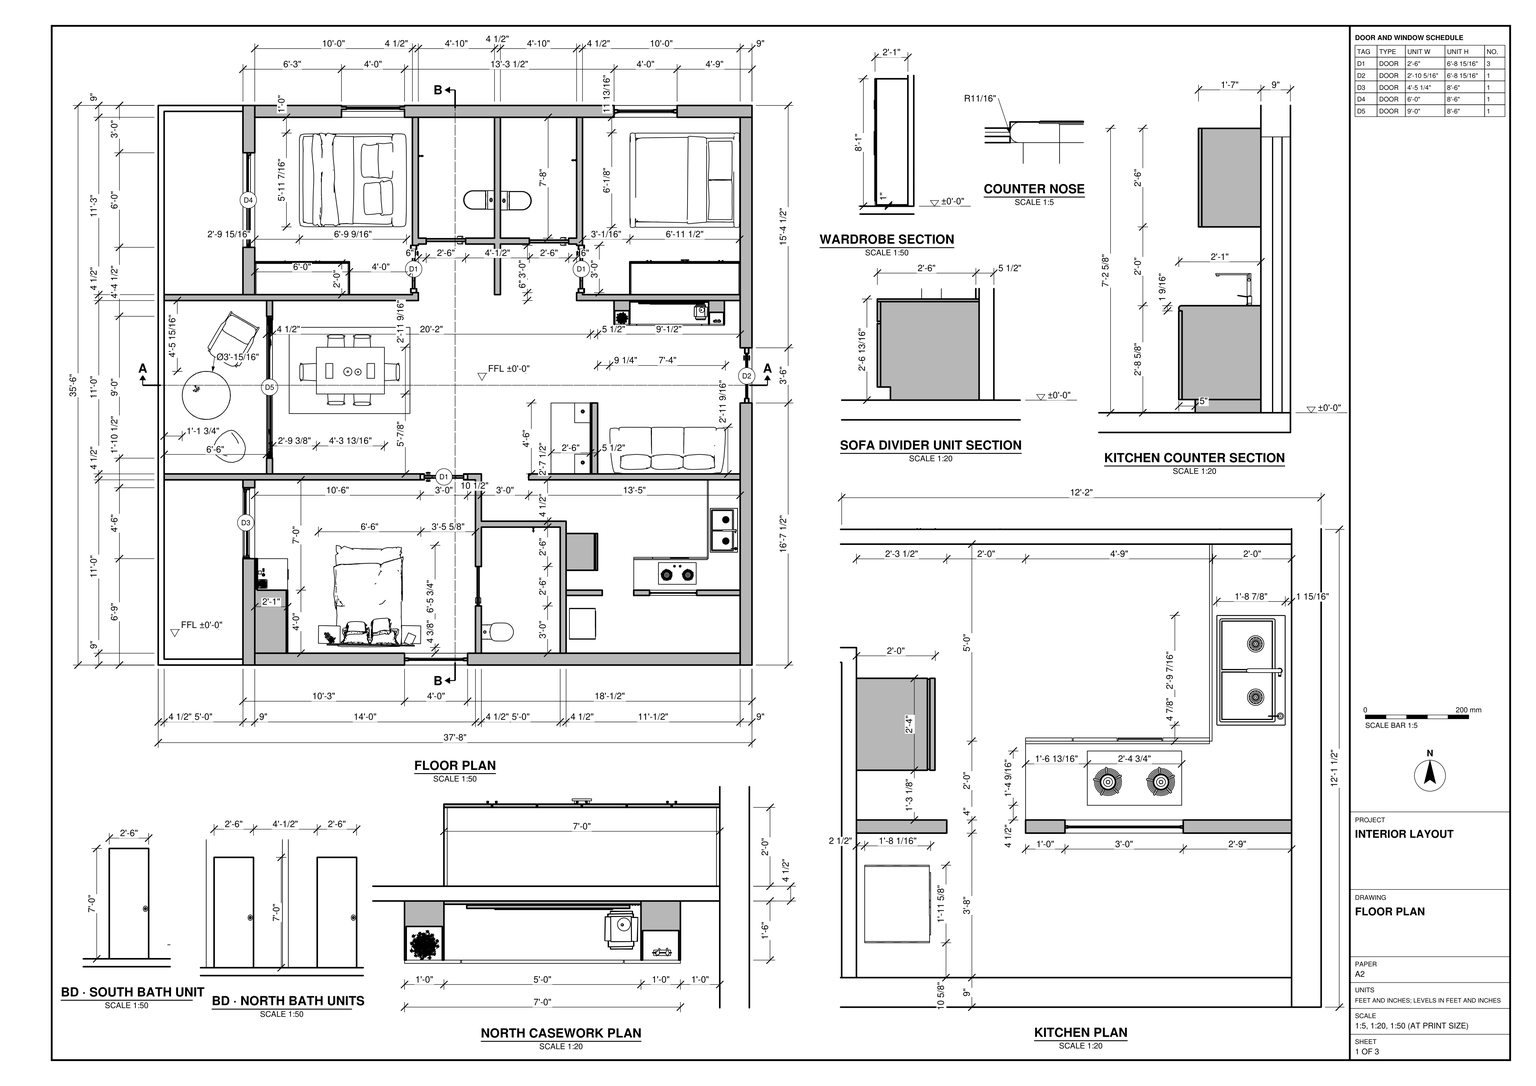
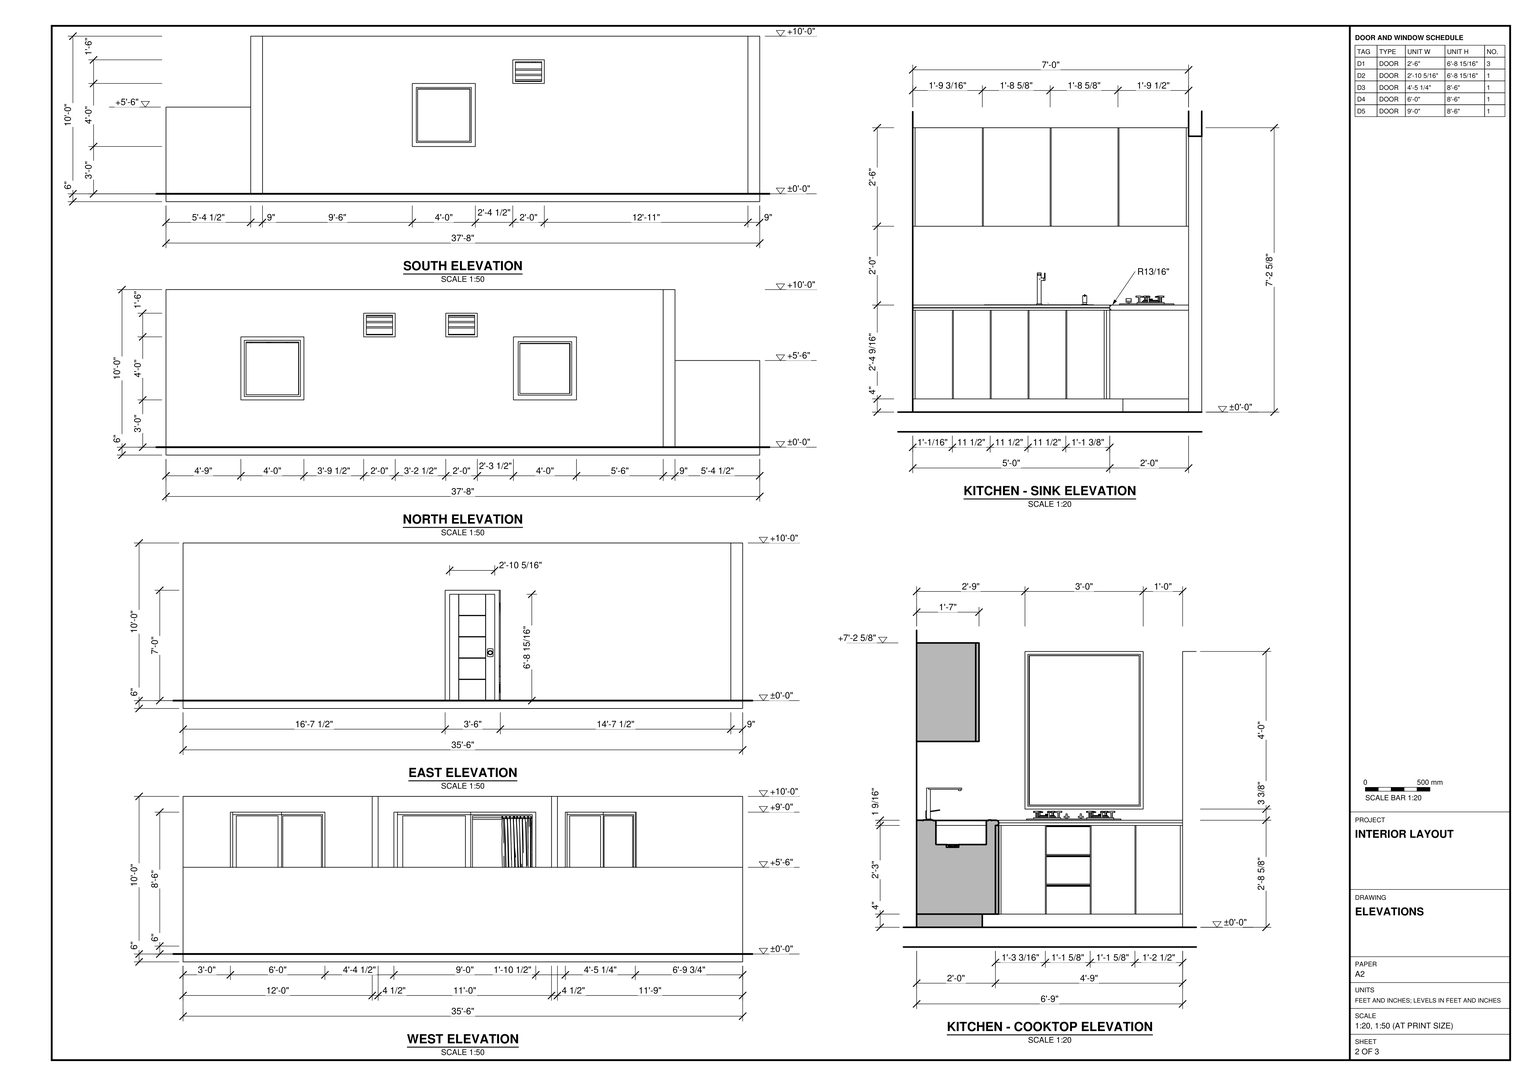
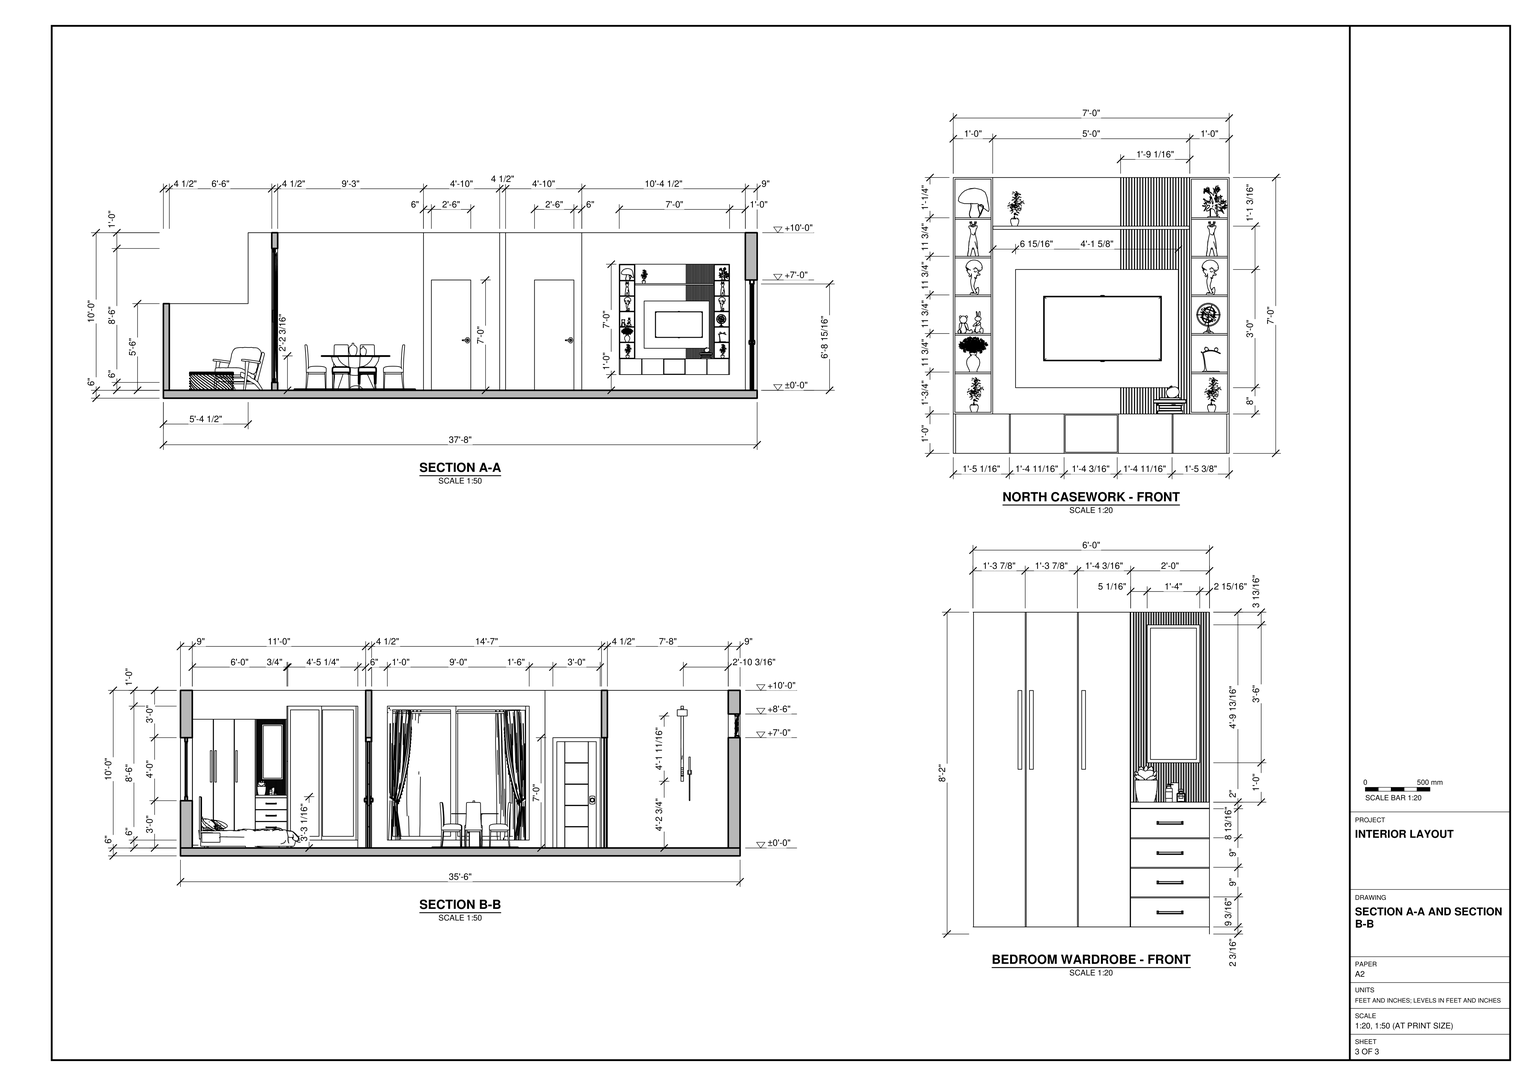
Build the residential interior in SketchUp from task_files/diagram_01.pdf. Work in feet and inches. Set the single finished floor at ±0'-0". The overall model shall measure 37'-8" east to west, 35'-6" north to south and 10'-6" from the underside of the slab to the top of the walls.

Use the floor plan to lay out the two north bedrooms and their paired bath units, the southwest bedroom with the adjoining bath unit, the central dining and living area, and the southeast kitchen. Include the west-side strip with its low perimeter wall and seating area. Model the floor slab, the 9" exterior walls and the 4 1/2" partitions where indicated. Use the elevations and sections to set wall heights and place the doors, glazed openings and high vents.

Fit out the rooms with beds, wardrobes, a dining table and chairs, and a sofa with its divider unit. Use the joinery details for the wardrobe fronts, the living-area display shelves and base cabinets, and the kitchen counters, upper cabinets, sink and cooktop. Decor and loose items may be any suitable library components, for example from 3D Warehouse.

Keep shell elements and each furniture or joinery piece in separate groups or components, and use components for repeated parts. Save one SketchUp model as output_files/furnished_three_bedroom_interior_with_built_in_joinery.skp.

# SketchUp Ruby script. Lengths in inches.
U = 1.inch
M = Sketchup.active_model
def pt(a) = Geom::Point3d.new(a.map { |v| v * U })
def face(e, loops, mat)
  f = e.add_face(loops[0].map { |a| pt(a) })
  loops[1..].each { |l| e.add_face(l.map { |a| pt(a) }).erase! }
  f.material = f.back_material = mat if mat
  f
end
# faces: each face lists its corners as indices into pts; further lists are holes
def faces(e, pts, list, mat = nil) = list.each { |f| face(e, (f[0].is_a?(Array) ? f : [f]).map { |l| l.map { |i| pts[i] } }, mat) }
# xy, xz, yz: faces in a plane at the given z, y or x. An outline is a flat list of corners, or four numbers for a rectangle; further outlines are holes
def ring(l) = l.size == 4 ? [[l[0], l[1]], [l[2], l[1]], [l[2], l[3]], [l[0], l[3]]] : l.each_slice(2).to_a
def flat(e, list, mat, &to3) = list.each { |f| face(e, (f[0].is_a?(Array) ? f : [f]).map { |l| ring(l).map { |u, v| to3.(u, v) } }, mat) }
def xy(e, z, list, mat = nil) = flat(e, list, mat) { |x, y| [x, y, z] }
def xz(e, y, list, mat = nil) = flat(e, list, mat) { |x, z| [x, y, z] }
def yz(e, x, list, mat = nil) = flat(e, list, mat) { |y, z| [x, y, z] }
def lines(e, pts, list) = list.each { |a, b| e.add_line(pt(pts[a]), pt(pts[b])) }
# prism: a flat outline (further loops are holes) pulled along v
def prism(e, loops, v, mat = nil)
  f = face(e, loops, mat); d = Geom::Vector3d.new(v.map { |x| x * U })
  f.pushpull(f.normal.samedirection?(d) ? d.length : -d.length)
end
def box(e, o, s, mat = nil) = prism(e, [[o, [o[0] + s[0], o[1], o[2]], [o[0] + s[0], o[1] + s[1], o[2]], [o[0], o[1] + s[1], o[2]]]], [0, 0, s[2]], mat)
def at(x, y, z, deg = 0) = Geom::Transformation.translation(pt([x, y, z])) * Geom::Transformation.rotation(ORIGIN, Z_AXIS, deg.degrees)
def axes(o, x, y, z) = Geom::Transformation.new([*x, 0, *y, 0, *z, 0, *pt(o).to_a, 1])
def part(name) = M.definitions.add(name)
# library, detail: a bought-in or finely detailed component or shape, given as its bounding box
def library(name, o, s) = part(name).tap { |d| box(d.entities, o, s) }
def detail(e, o, s) = box(e.add_group.entities, o, s)
def put(e, d, t, mat = nil) = e.add_instance(d, t).tap { |i| i.material = mat if mat }
def group(e, t, mat = nil) = e.add_group.tap { |g| g.transformation = t; g.material = mat if mat }.entities
root = M.entities
M.materials.add("Flooring Parquet Parallel E01 120cm").color = [119, 88, 63]
M.materials.add("Laminate C02 120cm").color = [189, 167, 139]
M.materials.add("MIRROR").color = [249, 248, 248]
M.materials["MIRROR"].alpha = 0.15
M.materials.add("Manhattan Creative Coating ML 1122B 24.81cm").color = [255, 255, 255]
M.materials.add("Marble 001 38.37cm").color = [255, 255, 255]
M.materials.add("Marble White 602 38.29cm").color = [255, 255, 255]
M.materials.add("Paint Blue Grain Matte 16.9cm").color = [255, 255, 255]
M.materials.add("Wood 13-11 100cm").color = [206, 162, 102]
M.materials.add("Wood Mahogany 33-46 100cm").color = [84, 42, 21]
M.materials.add("Wood Teak 33-35 100cm").color = [135, 81, 33]
M.materials.add("Wood Teak 33-35 100cm\#1").color = [135, 81, 33]
M.materials.add("[Carrera Marble]").color = [207, 207, 207]
M.materials.add("[Color A07]").color = [204, 180, 176]
M.materials.add("[Color M08]").color = [30, 30, 30]
M.materials.add("[Color M09]").color = [0, 0, 0]
M.materials.add("[Color_003]").color = [170, 170, 170]
M.materials.add("[Translucent Glass Gray]").color = [128, 128, 128]
M.materials["[Translucent Glass Gray]"].alpha = 0.5
M.materials.add("[Translucent Glass Sky Reflection]").color = [126, 138, 183]
M.materials["[Translucent Glass Sky Reflection]"].alpha = 0.52
M.materials.add("[Wood Bamboo]").color = [177, 105, 43]
M.materials.add("images").color = [98, 122, 106]
c1 = library("SLIDING+GLASS+DOOR",[0,-0.75,0],[72,5.75,80])
c2 = library("Untitled (14)",[0,0,0],[7.13,36,83])
c3 = library("Handle",[0,0,0],[0.66,1.27,5.34])
c4 = library("元件\#10",[0,0,0],[0.5625,0.71,6.64])
c5 = library("Cabinet bar pull",[0,0,0],[9.02,0.79,0.39])
c6 = library("Straight Handle",[-2.95,-1.38,-0.39],[5.9,1.38,0.78])
c7 = library("Bed 001",[-37.84,-46.07,0],[75.19,90.39,37.01])
c8 = library("Eva Bed",[-34.4,-44.85,0.04],[68.9,90.3,39.91])
c9 = library("Cabinet pull",[-0.17,-0.54,-0.33],[4.53,0.54,0.66])
c10 = part("Cabinet bar pull \#1")
xy(c10.entities,0,[[0,0,2,0.5]],"[Color M09]")
xy(c10.entities,0.4,[[0,0,1.4,0.5]],"[Color M09]")
xy(c10.entities,9.6,[[0,0,1.4,0.5]])
xy(c10.entities,10,[[0,0,2,0.5]],"[Color M09]")
xz(c10.entities,0,[[0,0,2,0,2,10,0,10,0,9.6,1.4,9.6,1.4,0.4,0,0.4]],"[Color M09]")
xz(c10.entities,0.5,[[0,0,0,0.4,1.4,0.4,1.4,9.6,0,9.6,0,10,2,10,2,0]],"[Color M09]")
yz(c10.entities,0,[[0,0,0.5,0.4],[0,9.6,0.5,10]])
yz(c10.entities,1.4,[[0,0.4,0.5,9.6]])
yz(c10.entities,2,[[0,0,0.5,10]],"[Color M08]")
c11 = library("Potted Plant 50-24",[-2.18,-2.1,0],[4.36,4.2,6.7])
c12 = library("Toiletry set",[28.69,-29.77,58.91],[5.39,6.58,5.91])
c13 = library("Curtains and rod",[2.63,-1.46,0.02],[153.32,14.02,114.15])
c14 = library("Mesa+de+Jantar+Clean-Ouro",[12.6875,-84.97,0.5625],[145.94,104.19,56.09])
c15 = library("Flat screen television",[0,1.41,1.14],[35.92,0.28,20.21])
c16 = library("6",[0,0,0],[30.12,28.16,55.56])
c17 = library("Decoration 111 063",[-2.51,-1.28,-0.03],[5.02,2.53,10.66])
c18 = library("Tree Decoration 83-10",[-18.61,-13.07,0],[43.1,29.04,44.77])
c19 = library("Decorative Figures 02 65-28",[-3.68,-1.82,0],[7.71,3.84,6.72])
c20 = library("Birds Figure 37-23",[-6.28,-2.57,0],[12.56,5.14,16.19])
c21 = library("Armillary Sphere 37-31",[-7.11,-7.1,0],[14.21,14.18,18.13])
c22 = library("Decorative Deer 209 004",[-1.58,-4.16,0],[3.36,7.25,10.63])
c23 = library("Vase Flowers 26-02",[-5.76,-5.9,0],[11.73,12.02,14.27])
c24 = library("Vase Flowers 63-21",[-12.07,-10.62,0],[22.87,22.48,21.95])
c25 = library("Books 155 025",[-5.0625,-5.83,0.01],[10.11,11.66,8.59])
c26 = library("Sofa 006",[-44,-16.57,0],[88,35.54,32.43])
c27 = library("Standing Toilet 84-06",[-6.89,-10.81,0],[13.78,24.43,31.08])
c28 = library("Shower Panel 127 022",[-3.8,-12.73,-35.99],[10.88,12.73,72])
c29 = library("Toilet",[-7.17,-23.62,0],[14.34,23.62,32.58])
c30 = library("Kitchen washbasin",[0,0,-0.81],[20.87,33.47,18.01])
c31 = library("Gas cooktop",[0,0,0],[16.54,28.74,2.76])
c32 = library("ENERGISK+B18+S (1)",[50,0,0],[28,31.125,68.4])
c33 = library("Component\#195",[0,0,0],[23.62,20.08,32.68])
c34 = library("Chair Lounge 009",[-13.99,-18.12,0],[27.98,36.23,32.73])
c35 = library("Table 291 011",[-29.63,-29.52,0],[59.27,59.05,22.03])
c36 = library("Lift Soft",[-11.58,-10.81,0],[23.13,23.73,30.98])
c37 = library("Flower pot",[0.35,0,0],[10.31,11.74,10.22])
c38 = library("Ganesha+-+An+Do+Giao",[8.43,-11.04,-0.14],[9.49,5.78,12.28])
c39 = library("Group\#24",[0,0,0],[6,36,80])
c40 = library("Group\#26",[0,0,0],[72,1,84])
c41 = library("Group\#38",[0,0,-2],[24,72,98])
c42 = library("ventilater",[0,0,0],[24,9,24])
c43 = library("Group\#41",[0,0,-2],[1,72,98])
c44 = library("Group\#43",[0,0,0],[1,24,36])
c45 = library("Group\#63",[-1.61,-2.52,0],[8.89,8.86,6.26])
c46 = library("Group\#65",[0,0,0],[4.43,4.97,6.14])
c47 = library("Group\#60",[0,-4.0625,0.24],[96.99,83.96,56.66])
c48 = library("Group\#74",[0,0,0],[81,84,31.02])
c49 = library("Group\#75",[0,0,0],[57,60,27.01])
c50 = library("Group\#79",[0,0,0],[1,84,30])
c51 = library("Group\#81",[-0.5,0,0],[132.5,4,120])
c52 = library("Group\#83",[0,0,0],[84,1,12])
c53 = part("Group\#86")
box(c53.entities,[0,0,0],[11,9,0.5])
c54 = part("Group\#87")
box(c54.entities,[0,0,0],[11,10.25,0.5])
c55 = library("Group\#37",[0,0,-1],[84,1,97])
c56 = part("Group\#89")
box(c56.entities,[0,0,0],[0.125,0.25,72])
c57 = library("Group\#76",[0,0,0],[81,84,1.57])
c58 = library("Group\#116",[0,0,0],[1,54,26])
box(root,[365.95,275.25,38],[49.61,1,36],"Marble 001 38.37cm")
xy(root,36.79,[[329,145.5,330,199.5]])
xy(root,51.79,[[317,145.5,329,160.5],[317,184.5,329,199.5]],"[Carrera Marble]")
xy(root,52.79,[[317,145.5,329,160.5],[317,184.5,329,199.5]],"[Carrera Marble]")
xy(root,76.79,[[317,145.5,329,160.5],[317,184.5,329,199.5]],"[Carrera Marble]")
xy(root,77.79,[[317,145.5,329,160.5],[317,184.5,329,199.5]],"[Carrera Marble]")
xy(root,101.79,[[317,145.5,329,160.5],[317,184.5,329,199.5]],"[Carrera Marble]")
xy(root,102.79,[[317,145.5,329,160.5],[317,184.5,329,199.5]],"[Carrera Marble]")
xy(root,120.79,[[329,145.5,330,199.5]])
xy(root,120.79,[[322,145.5,329,199.5]],"Wood Mahogany 33-46 100cm")
xy(root,121.79,[[322,145.5,330,199.5]],"Wood Mahogany 33-46 100cm")
xz(root,145.5,[[329,36.79,330,36.79,330,120.79,329,120.79,329,102.79,317,102.79,317,101.79,329,101.79,329,77.79,317,77.79,317,76.79,329,76.79,329,52.79,317,52.79,317,51.79,329,51.79],[322,120.79,330,121.79]])
xz(root,160.5,[[317,51.79,329,52.79],[317,76.79,329,77.79],[317,101.79,329,102.79]],"[Carrera Marble]")
xz(root,184.5,[[317,101.79,329,102.79]],"Wood Mahogany 33-46 100cm")
xz(root,184.5,[[317,51.79,329,52.79],[317,76.79,329,77.79]],"[Carrera Marble]")
xz(root,199.5,[[329,36.79,330,120.79],[322,120.79,330,121.79]],"Wood Mahogany 33-46 100cm")
xz(root,199.5,[[317,51.79,329,52.79],[317,76.79,329,77.79],[317,101.79,329,102.79]],"[Carrera Marble]")
xz(root,258.5,[[381.08,18.34,396.92,29.66]],"[Translucent Glass Sky Reflection]")
yz(root,317,[[145.5,51.79,160.5,52.79],[184.5,51.79,199.5,52.79],[145.5,76.79,160.5,77.79],[184.5,76.79,199.5,77.79],[145.5,101.79,160.5,102.79],
  [184.5,101.79,199.5,102.79]],"[Carrera Marble]")
yz(root,322,[[145.5,120.79,199.5,121.79]],"Wood Mahogany 33-46 100cm")
yz(root,329,[[184.5,51.79,199.5,52.79],[184.5,76.79,199.5,77.79],[184.5,101.79,199.5,102.79]])
yz(root,329,[[160.5,36.79,184.5,120.79]],"Manhattan Creative Coating ML 1122B 24.81cm")
yz(root,329,[[145.5,36.79,160.5,51.79],[184.5,36.79,199.5,51.79],[145.5,52.79,160.5,76.79],[184.5,52.79,199.5,76.79],[145.5,77.79,160.5,101.79],
  [184.5,77.79,199.5,101.79],[145.5,102.79,160.5,120.79],[184.5,102.79,199.5,120.79]],"Wood Mahogany 33-46 100cm")
yz(root,330,[[145.5,36.79,199.5,120.79]])
p = [[84.75,265.5,12],[84.75,157.5,12],[84.75,157.5,114],[84.75,265.5,114],[374,55,42],[410,55,42],
  [410,55,90],[374,55,90]]
lines(root,p,[[0,1],[1,2],[2,3],[3,0],[4,5],[5,6],[6,7],[7,4]])
put(root,c1,axes([83.09,265.5,12],[0,-1.5,0],[0.78261,0,0],[0,0,1.275]))
put(root,c1,axes([67.3,390,12],[0,-1,0],[0.59,0,0],[0,0,1.275]))
put(root,c1,axes([64.5,135,12],[0,-0.74,0],[1,0,0],[0,0,1.275]))
put(root,c2,axes([190.87,283.5,6],[1,0,0],[0,1,0],[0,0,1.01205]))
put(root,c2,axes([318.5,283.5,6],[1,0,0],[0,1,0],[0,0,1.01205]))
put(root,c2,axes([450.42,199.5,6],[-0.67534,0,0],[0,1.14416,0],[0,0,1.01205]))
put(root,c3,axes([128.35,308.61,71.08],[1,0,0],[0,-0.99808,-0.06194],[0,-0.06194,0.99808]))
put(root,c3,axes([125.85,308.61,71.08],[1,0,0],[0,-0.99808,-0.06194],[0,-0.06194,0.99808]))
put(root,c3,axes([92.32,308.61,71.08],[1,0,0],[0,-0.99808,-0.06194],[0,-0.06194,0.99808]))
put(root,c3,axes([90.07,308.61,71.08],[1,0,0],[0,-0.99808,-0.06194],[0,-0.06194,0.99808]))
put(root,c4,at(401.87,307,79.52))
put(root,c4,at(399.5,307,79.52))
put(root,c4,at(374.82,307,79.66))
put(root,c4,at(372.2,307,79.66))
put(root,c5,axes([429.41,307,63],[0,0,-1.99651],[0,1,0],[1,0,0]))
put(root,c5,axes([426.86,307,63],[0,0,-1.99651],[0,1,0],[1,0,0]))
put(root,c5,axes([402.16,307.1,63],[0,0,-1.99651],[0,1,0],[1,0,0]))
put(root,c5,axes([399.39,307,63],[0,0,-1.99651],[0,1,0],[1,0,0]))
put(root,c5,axes([374.75,307,63],[0,0,-1.99651],[0,1,0],[1,0,0]))
put(root,c5,axes([372.12,307,63],[0,0,-1.99651],[0,1,0],[1,0,0]))
put(root,c6,axes([401,307.23,27],[1,0,0],[0,-1,0],[0,0,1]))
put(root,c6,axes([401,307.23,15.3125],[1,0,0],[0,-1,0],[0,0,1]))
put(root,c7,axes([148.99,369.05,6],[0,-0.95,0],[0.9025,0,0],[0,0,0.95]))
put(root,c8,axes([400.375,369.05,6.47],[0.00004,-1.04495,0.00511],[0.92234,0,-0.00751],[0.00814,0.00489,0.99995]))
put(root,c9,axes([98.5,65.31,39.84],[0,1.76591,0],[-1,0,0],[0,0,1.44]))
put(root,c9,axes([98.5,65.31,30.66],[0,1.76591,0],[-1,0,0],[0,0,1.44]))
put(root,c9,axes([98.5,65.31,21.71],[0,1.76591,0],[-1,0,0],[0,0,1.44]))
put(root,c9,axes([98.5,65.31,12.58],[0,1.76591,0],[-1,0,0],[0,0,1.44]))
put(root,c10,axes([98.5,22.71,56.16],[1,0,0],[0,2.31,0],[0,0,2.4]))
put(root,c10,axes([98.5,26.21,56.16],[1,0,0],[0,2.31,0],[0,0,2.4]))
put(root,c10,axes([98.5,42.1,56.16],[1,0,0],[0,2.31,0],[0,0,2.4]))
put(root,c11,axes([79.49,61.61,46.16],[1.66,0,0],[0,1.66,0],[0,0,1.66]))
put(root,c12,at(47.49,96.97,-12.75))
put(root,c13,axes([86.67,155.65,5.98],[0,0.70441,0],[-0.2234,0,0],[0,0,0.94608]))
put(root,c14,axes([91.69,244.99,6.21],[0.63,0,0],[0,0.63,0],[0,0,0.63]))
put(root,c4,at(429.49,307,80))
put(root,c4,at(426.68,307,80))
put(root,c15,at(374.47,273.5625,44.78))
put(root,c16,axes([422.83,261.83,30.5],[0.19,0,0],[0,0.19,0],[0,0,0.19]))
put(root,c16,axes([350.52,261.83,30.5],[0.19,0,0],[0,0.19,0],[0,0,0.19]))
put(root,c16,axes([362.86,266.83,87.2],[0.19,0,0],[0,0.19,0],[0,0,0.19]))
put(root,c17,at(353.32,263.55,66.25))
put(root,c17,at(425.23,264.47,66.25))
put(root,c18,axes([426.27,262.39,89.75],[0.18343,0,0],[0,0.221,0],[0,0,0.221]))
put(root,c19,at(352.0625,262.875,54.5))
put(root,c20,axes([425.39,261.92,42.75],[0.47,0,0],[0,0.47,0],[0,0,0.47]))
put(root,c21,axes([424.68,263.12,54.5],[0.51,0,0],[0,0.51,0],[0,0,0.51]))
put(root,c22,at(425.63,262.88,78))
put(root,c22,at(352.93,264.83,78))
put(root,c23,axes([353.06,263.99,42.75],[0.76,0,0],[0,0.76,0],[0,0,0.76]))
put(root,c24,axes([353.47,263.85,89.75],[0.41,0,0],[0,0.41,0],[0,0,0.41]))
put(root,c25,at(413.01,268.63,30))
put(root,c16,axes([391.23,260.41,18.34],[0.19,0,0],[0,0.19,0],[0,0,0.19]))
put(root,c26,at(387.75,164.47,6,180))
put(root,c27,at(259.62,25.14,16.64,90))
put(root,c28,at(280,105,78.34))
put(root,c29,axes([256,354.0625,12.14],[0,1,0],[1,0,0],[0,0,1]))
put(root,c29,axes([260.5,353.52,17.89],[0,-1,0],[-1,0,0],[0,0,1]))
put(root,c30,at(441.08,119.32,31.2,-180))
put(root,c31,at(409.53,61.47,38.6,90))
put(root,c32,axes([334.5,22.15,6],[0,1,0],[-0.77108,0,0],[0,0,1]))
put(root,c33,at(333.08,19.61,6,90))
put(root,c34,at(57.08,247.33,6,-30))
put(root,c35,axes([36.6,205.28,6],[0.62,0,0],[0,0.62,0],[0,0,0.62]))
put(root,c36,at(54.26,166.1875,6,-132.1))
put(root,c16,axes([26.18,207.6,19.66],[0.19,0,0],[0,0.19,0],[0,0,0.19]))
put(root,c16,axes([320.33,190.39,52.79],[0.19,0,0],[0,0.19,0],[0,0,0.19]))
put(root,c16,axes([320.33,151.51,52.79],[0.19,0,0],[0,0.19,0],[0,0,0.19]))
put(root,c37,at(317.74,185.94,102.79))
put(root,c37,at(317.74,146.94,102.79))
put(root,c38,at(331.55,205.47,77.93,-90))
put(root,c38,at(331.55,165.28,77.93,-90))
put(root,c28,at(198,381.97,77.99,90))
put(root,c28,at(318.5,389.9,77.99,-90))
g1 = group(root,at(64.5,0,0))
box(g1,[-64.5,0,0],[452,426,6])
g2 = group(root,at(64.5,0,6))
xy(g2,0,[[0,0,9,81],[0,81,9,135],[0,135,9,141],[0,282,9,318],[0,318,9,390],
  [0,390,9,426]])
xy(g2,6,[[0,81,9,135],[0,318,9,390]])
xy(g2,108,[[0,81,9,135],[0,318,9,390]])
xy(g2,120,[[0,0,9,141],[0,282,9,426]])
xz(g2,0,[[0,0,9,120]])
xz(g2,81,[[0,0,9,6],[0,6,9,108]])
xz(g2,135,[[0,0,9,6],[0,6,9,108]])
xz(g2,141,[[0,0,9,120]])
xz(g2,282,[[0,0,9,120]])
xz(g2,318,[[0,0,9,6],[0,6,9,108]])
xz(g2,390,[[0,0,9,6],[0,6,9,108]])
xz(g2,426,[[0,0,9,120]])
yz(g2,0,[[0,0,0,120,141,120,141,0,135,0,135,108,81,108,81,0],[81,0,135,6],[282,0,282,120,426,120,426,0,390,0,390,108,318,108,318,0],[318,0,390,6]])
yz(g2,9,[[0,0,81,0,81,108,135,108,135,0,141,0,141,120,0,120],[81,0,135,6],[282,0,318,0,318,108,390,108,390,0,426,0,426,120,282,120],[318,0,390,6]])
g3 = group(root,at(311,141,6))
box(g3,[-29,0,0],[161,4.5,120])
g4 = group(root,at(82.5,145.5,6))
prism(g4,[[[4.5,12,0],[4.5,120,0],[4.5,132,0],[4.5,132,120],[4.5,0,120],[4.5,0,0]],[[4.5,120,108],[4.5,120,6],[4.5,12,6],[4.5,12,108]]],[-4.5,0,0])
g5 = group(root,at(0,0,6))
prism(g5,[[[64.5,0,0],[0,0,0],[0,426,0],[64.5,426,0],[64.5,421.5,0],[4.5,421.5,0],[4.5,4.5,0],[64.5,4.5,0]]],[0,0,66])
put(root,c39,axes([234,320.5,6],[0,1,0],[-0.83333,0,0],[0,0,1.05]))
put(root,c39,axes([312.5,319.5,6],[0,1,0],[-0.83333,0,0],[0,0,1.05]))
g6 = group(root,at(73.5,282,7))
prism(g6,[[[1,0,0],[71,0,0],[71,0,-1],[72,0,-1],[72,0,84],[0,0,84],[0,0,-1],[1,0,-1]]],[0,24,0],"Wood Teak 33-35 100cm")
put(root,c40,at(73.5,306,7))
put(root,c41,at(73.5,9,8),"Paint Blue Grain Matte 16.9cm")
g7 = group(root,at(4.5,9,6))
put(g7,c2,axes([231,130.69,0],[0,1,0],[-1,0,0],[0,0,1.01205]))
g8 = group(g7,at(69,0,0))
xy(g8,0,[[232.5,0,232.5,96,172.5,96,172.5,66,168,66,168,132,162,132,162,136.5,172.5,136.5,172.5,100.5,237,100.5,237,0],[168,0,172.5,36],[-69,132,126,136.5]])
xy(g8,66,[[-69,132,-9,136.5]])
xy(g8,84,[[168,36,172.5,66],[126,132,162,136.5]])
xy(g8,120,[[168,0,172.5,0,172.5,96,232.5,96,232.5,0,237,0,237,100.5,172.5,100.5,172.5,136.5,-9,136.5,-9,132,168,132]])
xz(g8,0,[[168,0,172.5,120],[232.5,0,237,120]])
xz(g8,36,[[168,0,172.5,84]])
xz(g8,66,[[168,0,172.5,84]])
xz(g8,96,[[172.5,0,232.5,120]])
xz(g8,100.5,[[172.5,0,237,120]])
xz(g8,132,[[-69,0,126,0,126,84,162,84,162,0,168,0,168,120,-9,120,-9,66,-69,66]])
xz(g8,136.5,[[-69,0,-69,66,-9,66,-9,120,172.5,120,172.5,0,162,0,162,84,126,84,126,0]])
yz(g8,-69,[[132,0,136.5,66]])
yz(g8,-9,[[132,66,136.5,120]])
yz(g8,126,[[132,0,136.5,84]])
yz(g8,162,[[132,0,136.5,84]])
yz(g8,168,[[0,0,0,120,132,120,132,0,66,0,66,84,36,84,36,0]])
yz(g8,172.5,[[0,0,36,0,36,84,66,84,66,0,96,0,96,120,0,120],[100.5,0,136.5,120]])
yz(g8,232.5,[[0,0,96,120]])
yz(g8,237,[[0,0,100.5,120]])
put(g7,c39,axes([237,36,0],[0.67633,0,0],[0,0.83333,0],[0,0,1.05]))
g9 = group(root,at(73.5,0,6))
xy(g9,36,[[114,3.4,162,4.5],[114,4.5,162,5.27]])
xy(g9,39.0625,[[117.0625,3.4,158.9375,3.9],[117.0625,4.65,158.9375,5.27]])
xy(g9,40.0625,[[118.0625,3.9,157.9375,4.65]])
xy(g9,79.9375,[[118.0625,3.9,157.9375,4.65]])
xy(g9,80.9375,[[117.0625,3.4,158.9375,3.9],[117.0625,4.65,158.9375,5.27]])
xy(g9,84,[[114,3.4,162,4.5],[114,4.5,162,5.27]])
xz(g9,3.4,[[[114,36,162,84],[117.0625,39.0625,158.9375,80.9375]]])
xz(g9,3.9,[[[117.0625,39.0625,158.9375,80.9375],[118.0625,40.0625,157.9375,79.9375]]])
xz(g9,4.65,[[[117.0625,39.0625,158.9375,80.9375],[118.0625,40.0625,157.9375,79.9375]]])
xz(g9,5.27,[[[114,36,162,84],[117.0625,39.0625,158.9375,80.9375]]])
yz(g9,114,[[3.4,36,4.5,84],[4.5,36,5.27,84]])
yz(g9,117.0625,[[3.4,39.0625,3.9,80.9375],[4.65,39.0625,5.27,80.9375]])
yz(g9,118.0625,[[3.9,40.0625,4.65,79.9375]])
yz(g9,157.9375,[[3.9,40.0625,4.65,79.9375]])
yz(g9,158.9375,[[3.4,39.0625,3.9,80.9375],[4.65,39.0625,5.27,80.9375]])
yz(g9,162,[[3.4,36,4.5,84],[4.5,36,5.27,84]])
p = [[118.0625,4.33,79.68],[118.0625,4.33,40.0625],[157.8,4.24,40.0625],[157.8,4.24,79.68]]
faces(g9,p,[[0,1,2,3]],"[Translucent Glass Gray]")
put(g9,c42,axes([190.5,1.61,84],[1,0,0],[0,0.34295,0],[0,0,0.75]))
put(g9,c5,axes([49.1,307,37.16],[0,0,-1.331],[0,1,0],[1,0,0]))
put(g9,c5,axes([46.43,307,37.16],[0,0,-1.331],[0,1,0],[1,0,0]))
put(g9,c5,axes([22.87,307,37.16],[0,0,-1.331],[0,1,0],[1,0,0]))
g10 = group(g9,at(0,0,0))
prism(g10,[[[369.5,9,0],[0,9,0],[0,9,120],[369.5,9,120]],[[114,9,84],[114,9,36],[162,9,36],[162,9,84]],[[214.5,9,102],[190.5,9,102],[190.5,9,84],[214.5,9,84]]],[0,-9,0])
put(root,c43,at(97.5,9,8))
g11 = group(root,at(75.5,57,8.16))
prism(g11,[[[0,0,0],[22,0,0],[22,0,36],[22,0,36.16],[23,0,36.16],[23,0,38],[0,0,38]]],[0,24,0],"Laminate C02 120cm")
put(root,c44,at(97.5,57,8.16))
g12 = group(root,at(75.5,62.04,58.16))
xy(g12,0,[[0,0,0.8125,16]])
xy(g12,1,[[0.5625,1,0.8125,15]])
xy(g12,41,[[0.5625,1,0.8125,15]])
xy(g12,42,[[0,0,0.8125,16]])
xz(g12,0,[[0,0,0.8125,42]])
xz(g12,1,[[0.5625,1,0.8125,41]])
xz(g12,15,[[0.5625,1,0.8125,41]])
xz(g12,16,[[0,0,0.8125,42]])
yz(g12,0,[[0,0,16,42]])
yz(g12,0.5625,[[1,1,15,41]],"MIRROR")
yz(g12,0.8125,[[[0,0,16,42],[1,1,15,41]]])
put(root,c45,axes([133.75,22.07,19.625],[-1.01425,-0.29659,0],[0.29677,-1.01488,0],[0,0,0.86321]))
put(root,c46,axes([130.41,25.8,19.625],[-1.01425,-0.29659,0],[0.29677,-1.01488,0],[0,0,0.86321]))
g13 = group(root,at(187.21,14.86,17.16),"[Color A07]")
p = [[3.33,9.67,0.23],[8.88,7.25,0],[5.55,0,0.1],[0,2.42,0.32],[8.9,7.25,0.26],[5.57,0,0.36],
  [3.34,9.67,0.48],[0.01,2.42,0.58]]
faces(g13,p,[[0,1,2,3],[2,1,4,5],[1,0,6,4],[3,2,5,7],[0,3,7,6]],"[Color_003]")
faces(g13,p,[[4,6,7,5]],"images")
put(root,c47,axes([121.91,13.39,5.83],[0.80419,0,0],[0,0.99638,0],[0,0,0.69]),"[Color A07]")
put(root,c48,at(362,57,6))
put(root,c49,at(362,81,10.02))
g14 = group(root,at(425,57,62.6),"[Wood Bamboo]")
box(g14,[0,0,0],[18,84,30],"Wood 13-11 100cm")
put(root,c50,at(424,57,62.6),"Wood 13-11 100cm")
put(root,c51,at(311,53,6))
g15 = group(root,at(347,259.5,18))
xy(g15,0,[[0,0,84,18]],"Wood Teak 33-35 100cm\#1")
xy(g15,0.34,[[34.08,0,49.92,9]],"Wood Teak 33-35 100cm\#1")
xy(g15,11.66,[[34.08,0,49.92,9]],"Wood Teak 33-35 100cm\#1")
xy(g15,12,[[0,0,84,18]],"Wood Teak 33-35 100cm\#1")
xz(g15,0,[[[0,0,84,12],[34.08,0.34,49.92,11.66]]],"Wood Teak 33-35 100cm\#1")
xz(g15,9,[[34.08,0.34,49.92,11.66]],"Wood Teak 33-35 100cm\#1")
xz(g15,18,[[0,0,84,12]],"Wood Teak 33-35 100cm\#1")
yz(g15,0,[[0,0,18,12]],"Wood Teak 33-35 100cm\#1")
yz(g15,34.08,[[0,0.34,9,11.66]],"Wood Teak 33-35 100cm\#1")
yz(g15,49.92,[[0,0.34,9,11.66]],"Wood Teak 33-35 100cm\#1")
yz(g15,84,[[0,0,18,12]],"Wood Teak 33-35 100cm\#1")
put(root,c52,at(347,258.5,18))
g16 = group(root,at(419,259.5,30),"Wood Teak 33-35 100cm\#1")
xy(g16,0,[[0,0,12,18]])
xy(g16,0.5,[[0.5,0,11.5,9]])
xy(g16,71.5,[[0.5,0,11.5,9]])
xy(g16,72,[[0,0,12,18]])
xz(g16,0,[[[0,0,12,72],[0.5,0.5,11.5,71.5]]])
xz(g16,9,[[0.5,0.5,11.5,71.5]])
xz(g16,18,[[0,0,12,72]])
yz(g16,0,[[0,0,18,72]])
yz(g16,0.5,[[0,0.5,9,71.5]])
yz(g16,11.5,[[0,0.5,9,71.5]])
yz(g16,12,[[0,0,18,72]])
g17 = group(root,at(347,259.5,30),"Wood Teak 33-35 100cm\#1")
xy(g17,0,[[0,0,12,18]])
xy(g17,0.5,[[0.5,0,11.5,10.25]])
xy(g17,71.5,[[0.5,0,11.5,10.25]])
xy(g17,72,[[0,0,12,18]])
xz(g17,0,[[[0,0,12,72],[0.5,0.5,11.5,71.5]]])
xz(g17,10.25,[[0.5,0.5,11.5,71.5]])
xz(g17,18,[[0,0,12,72]])
yz(g17,0,[[0,0,18,72]])
yz(g17,0.5,[[0,0.5,10.25,71.5]])
yz(g17,11.5,[[0,0.5,10.25,71.5]])
yz(g17,12,[[0,0,18,72]])
put(root,c53,at(419.5,259.5,42.25),"Wood Teak 33-35 100cm\#1")
put(root,c53,at(419.5,259.5,54),"Wood Teak 33-35 100cm\#1")
put(root,c53,at(419.5,259.5,65.75),"Wood Teak 33-35 100cm\#1")
put(root,c53,at(419.5,259.5,77.5),"Wood Teak 33-35 100cm\#1")
put(root,c53,at(419.5,259.5,89.25),"Wood Teak 33-35 100cm\#1")
put(root,c54,at(347.5,259.5,42.25),"Wood Teak 33-35 100cm\#1")
put(root,c54,at(347.5,259.5,54),"Wood Teak 33-35 100cm\#1")
put(root,c54,at(347.5,259.5,65.75),"Wood Teak 33-35 100cm\#1")
put(root,c54,at(347.5,259.5,77.5),"Wood Teak 33-35 100cm\#1")
put(root,c54,at(347.5,259.5,89.25),"Wood Teak 33-35 100cm\#1")
g18 = group(root,at(359,276.5,30))
xy(g18,0,[[0,0,60,1]])
xy(g18,72,[[0,0,60,1]])
xz(g18,0,[[38.9375,0,60,72]])
xz(g18,0,[[0,0,38.9375,72]],"Marble White 602 38.29cm")
xz(g18,1,[[0,0,60,72]])
yz(g18,0,[[0,0,1,72]])
yz(g18,60,[[0,0,1,72]])
put(root,c55,at(359,306,7))
g19 = group(root,at(443,0,6))
prism(g19,[[[9,0,0],[9,199.5,0],[9,199.5,84],[9,241.5,84],[9,241.5,0],[9,417,0],[9,417,120],[9,0,120]]],[-9,0,0])
g20 = group(root,at(73.5,277.5,6))
xy(g20,0,[[-69,0,-69,4.5,120,4.5,120,6,124.5,6,124.5,0],[245,0,245,6,249.5,6,249.5,4.5,369.5,4.5,369.5,0],[182.5,4.5,182.5,43,160.5,43,160.5,47.5,182.5,47.5,182.5,139.5,187,139.5,187,47.5,209,47.5,209,43,187,43,187,4.5],[120,42,120,139.5,124.5,139.5,124.5,47.5,130.5,47.5,130.5,43,124.5,43,124.5,42],[245,42,245,43,239,43,239,47.5,245,47.5,245,139.5,249.5,139.5,249.5,42]])
xy(g20,66,[[-69,0,-9,4.5]])
xy(g20,84,[[120,6,124.5,42],[245,6,249.5,42],[130.5,43,160.5,47.5],[209,43,239,47.5]])
xy(g20,120,[[-9,0,124.5,0,124.5,43,182.5,43,182.5,4.5,187,4.5,187,43,249.5,43,249.5,139.5,245,139.5,245,47.5,187,47.5,187,139.5,182.5,139.5,182.5,47.5,124.5,47.5,124.5,139.5,120,139.5,120,4.5,-9,4.5],[245,0,369.5,0,369.5,4.5,249.5,4.5,249.5,43,245,43]])
xz(g20,0,[[-69,0,124.5,0,124.5,120,-9,120,-9,66,-69,66],[245,0,369.5,120]])
xz(g20,4.5,[[-69,0,-69,66,-9,66,-9,120,120,120,120,0],[182.5,0,187,120],[249.5,0,369.5,120]])
xz(g20,6,[[120,0,124.5,84],[245,0,249.5,84]])
xz(g20,42,[[120,0,124.5,84],[245,0,249.5,84]])
xz(g20,43,[[124.5,0,130.5,0,130.5,84,160.5,84,160.5,0,182.5,0,182.5,120,124.5,120],[187,0,209,0,209,84,239,84,239,0,245,0,245,120,187,120]])
xz(g20,47.5,[[124.5,0,124.5,120,182.5,120,182.5,0,160.5,0,160.5,84,130.5,84,130.5,0],[187,0,187,120,245,120,245,0,239,0,239,84,209,84,209,0]])
xz(g20,139.5,[[120,0,124.5,120],[182.5,0,187,120],[245,0,249.5,120]])
yz(g20,-69,[[0,0,4.5,66]])
yz(g20,-9,[[0,66,4.5,120]])
yz(g20,120,[[4.5,0,4.5,120,139.5,120,139.5,0,42,0,42,84,6,84,6,0]])
yz(g20,124.5,[[0,0,6,0,6,84,42,84,42,0,43,0,43,120,0,120],[47.5,0,139.5,120]])
yz(g20,130.5,[[43,0,47.5,84]])
yz(g20,160.5,[[43,0,47.5,84]])
yz(g20,182.5,[[4.5,0,43,120],[47.5,0,139.5,120]])
yz(g20,187,[[4.5,0,43,120],[47.5,0,139.5,120]])
yz(g20,209,[[43,0,47.5,84]])
yz(g20,239,[[43,0,47.5,84]])
yz(g20,245,[[0,0,0,120,43,120,43,84,6,84,6,0],[42,0,43,84],[47.5,0,139.5,120]])
yz(g20,249.5,[[4.5,0,6,0,6,84,42,84,42,0,139.5,0,139.5,120,4.5,120]])
yz(g20,369.5,[[0,0,4.5,120]])
p = [[245,43,84],[249.5,43,84]]
lines(g20,p,[[0,1]])
g21 = group(root,at(359,282,7))
xy(g21,-1,[[83,0,84,24]])
xy(g21,-0.9375,[[0,0,1,24]])
xy(g21,0,[[1,0,83,24]])
xy(g21,96,[[0,0,84,24]],"Flooring Parquet Parallel E01 120cm")
xz(g21,0,[[83,-1,84,-1,84,96,0,96,0,-0.9375,1,-0.9375,1,0,83,0]])
xz(g21,24,[[83,-1,83,3,1,3,1,-0.9375,0,-0.9375,0,96,84,96,84,-1]])
xz(g21,24,[[1,0,83,3]],"Flooring Parquet Parallel E01 120cm")
yz(g21,0,[[0,-0.9375,24,96]],"Flooring Parquet Parallel E01 120cm")
yz(g21,1,[[0,-0.9375,24,0]])
yz(g21,83,[[0,-1,24,0]])
yz(g21,84,[[0,-1,24,96]])
g22 = group(root,at(73.5,282,6))
put(g22,c42,axes([141.5,140.25,84],[1,0,0],[0,0.29494,0],[0,0,0.75]))
put(g22,c42,axes([204,136.8,84],[1,0,0],[0,0.34295,0],[0,0,0.75]))
g23 = group(g22,at(0,0,0))
xy(g23,36,[[273.5,138.42,321.5,139.5],[273.5,139.5,321.5,140.73]])
xy(g23,38.625,[[276.125,138.42,318.875,139.08],[276.125,140.08,318.875,140.73]])
xy(g23,39.9375,[[277.4375,139.08,317.5625,140.08]])
xy(g23,80.0625,[[277.4375,139.08,317.5625,140.08]])
xy(g23,81.375,[[276.125,138.42,318.875,139.08],[276.125,140.08,318.875,140.73]])
xy(g23,84,[[273.5,138.42,321.5,139.5],[273.5,139.5,321.5,140.73]])
xz(g23,138.42,[[[273.5,36,321.5,84],[276.125,38.625,318.875,81.375]]])
xz(g23,139.08,[[[276.125,38.625,318.875,81.375],[277.4375,39.9375,317.5625,80.0625]]])
yz(g23,273.5,[[138.42,36,139.5,84],[139.5,36,140.73,84]])
yz(g23,276.125,[[138.42,38.625,139.08,81.375],[140.08,38.625,140.73,81.375]])
yz(g23,277.4375,[[139.08,39.9375,140.08,80.0625]])
yz(g23,317.5625,[[139.08,39.9375,140.08,80.0625]])
yz(g23,318.875,[[138.42,38.625,139.08,81.375],[140.08,38.625,140.73,81.375]])
yz(g23,321.5,[[138.42,36,139.5,84],[139.5,36,140.73,84]])
p = [[285.5,24,0],[285.5,0,0]]
lines(g23,p,[[0,1]])
g24 = group(g23,at(0,135,0))
xz(g24,5.08,[[[276.125,38.625,318.875,81.375],[277.4375,39.9375,317.5625,80.0625]]])
xz(g24,5.73,[[[273.5,36,321.5,84],[276.125,38.625,318.875,81.375]]])
g25 = group(g24,at(0,0,0))
xz(g25,4.51,[[277.62,39.9375,317.5625,79.46]],"[Translucent Glass Gray]")
g26 = group(g25,at(0,0,0))
p = [[109.11,6.8,40.89],[71.22,6.98,40.89],[71.22,6.98,78.79],[109.11,6.8,78.79]]
faces(g26,p,[[0,1,2,3]],"[Translucent Glass Gray]")
g27 = group(g26,at(0,0,0))
xy(g27,0,[[0,0,378.5,9]])
xy(g27,36,[[66,0,114,4.5],[273.5,0,321.5,9],[66,4.5,114,6.06],[66,7.99,114,9]])
xy(g27,39.64,[[69.64,6.06,110.36,6.53],[69.64,7.46,110.36,7.99]])
xy(g27,40.89,[[70.89,6.53,109.11,7.46]])
xy(g27,79.11,[[70.89,6.53,109.11,7.46]])
xy(g27,80.36,[[69.64,6.06,110.36,6.53],[69.64,7.46,110.36,7.99]])
xy(g27,84,[[66,0,114,4.5],[141.5,0,165.5,9],[204,0,228,9],[273.5,0,321.5,9],[66,4.5,114,6.06],
  [66,7.99,114,9]])
xy(g27,102,[[141.5,0,165.5,9],[204,0,228,9]])
xy(g27,120,[[0,0,378.5,9]])
xz(g27,0,[[[0,0,378.5,120],[66,36,114,84],[273.5,36,321.5,84],[141.5,84,165.5,102],[204,84,228,102]]])
xz(g27,6.06,[[[66,36,114,84],[69.64,39.64,110.36,80.36]]])
xz(g27,6.53,[[[69.64,39.64,110.36,80.36],[70.89,40.89,109.11,79.11]]])
xz(g27,7.46,[[[69.64,39.64,110.36,80.36],[70.89,40.89,109.11,79.11]]])
xz(g27,7.99,[[[66,36,114,84],[69.64,39.64,110.36,80.36]]])
xz(g27,9,[[[0,0,378.5,120],[66,36,114,84],[273.5,36,321.5,84],[141.5,84,165.5,102],[204,84,228,102]]])
yz(g27,0,[[0,0,9,120]])
yz(g27,66,[[0,36,4.5,84],[4.5,36,6.06,84],[7.99,36,9,84]])
yz(g27,69.64,[[6.06,39.64,6.53,80.36],[7.46,39.64,7.99,80.36]])
yz(g27,70.89,[[6.53,40.89,7.46,79.11]])
yz(g27,109.11,[[6.53,40.89,7.46,79.11]])
yz(g27,110.36,[[6.06,39.64,6.53,80.36],[7.46,39.64,7.99,80.36]])
yz(g27,114,[[0,36,4.5,84],[4.5,36,6.06,84],[7.99,36,9,84]])
yz(g27,141.5,[[0,84,9,102]])
yz(g27,165.5,[[0,84,9,102]])
yz(g27,204,[[0,84,9,102]])
yz(g27,228,[[0,84,9,102]])
yz(g27,273.5,[[0,36,9,84]])
yz(g27,321.5,[[0,36,9,84]])
yz(g27,378.5,[[0,0,9,120]])
g28 = group(root,at(397.9375,276.25,30),"Wood Teak 33-35 100cm\#1")
g29 = group(g28,at(0,0.25,0))
box(g29,[0,-0.0625,0],[21.0625,0.0625,72])
put(g28,c56,at(0,0,0))
put(g28,c56,at(0.84,0,0))
put(g28,c56,at(1.68,0,0))
put(g28,c56,at(2.51,0,0))
put(g28,c56,at(3.35,0,0))
put(g28,c56,at(4.1875,0,0))
put(g28,c56,at(5.02,0,0))
put(g28,c56,at(5.86,0,0))
put(g28,c56,at(6.7,0,0))
put(g28,c56,at(7.54,0,0))
put(g28,c56,at(8.375,0,0))
put(g28,c56,at(9.21,0,0))
put(g28,c56,at(10.05,0,0))
put(g28,c56,at(10.89,0,0))
put(g28,c56,at(11.73,0,0))
put(g28,c56,at(12.5625,0,0))
put(g28,c56,at(13.4,0,0))
put(g28,c56,at(14.24,0,0))
put(g28,c56,at(15.07,0,0))
put(g28,c56,at(15.91,0,0))
put(g28,c56,at(16.75,0,0))
put(g28,c56,at(17.59,0,0))
put(g28,c56,at(18.43,0,0))
put(g28,c56,at(19.26,0,0))
put(g28,c56,at(20.1,0,0))
put(g28,c56,at(20.9375,0,0))
g30 = group(root,at(359.08,263.8125,86.2),"Wood Teak 33-35 100cm")
box(g30,[0,0,0],[59.79,12.4375,1])
put(root,c57,at(362,57,37.02))
g31 = group(root,at(330,145.5,6))
box(g31,[0,0,0],[4.5,54,120])
g32 = group(root,at(300,145.5,6),"[Carrera Marble]")
xy(g32,0,[[3,0,30,54]])
xy(g32,4,[[0,0,3,54]])
xy(g32,30,[[0,0,30,54]])
xz(g32,0,[[3,0,30,0,30,30,0,30,0,4,3,4]])
xz(g32,54,[[3,0,3,4,0,4,0,30,30,30,30,0]])
yz(g32,0,[[0,4,54,30]])
yz(g32,3,[[0,0,54,4]],"Wood Mahogany 33-46 100cm")
yz(g32,30,[[0,0,54,30]])
put(root,c58,at(299,145.5,10),"[Carrera Marble]")
g33 = group(root,at(300,145.5,36),"[Carrera Marble]")
box(g33,[-1,0,0],[31,54,0.79])
